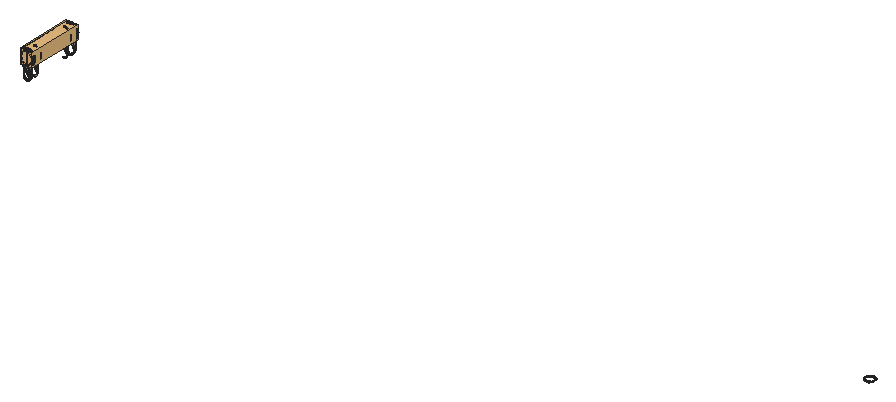
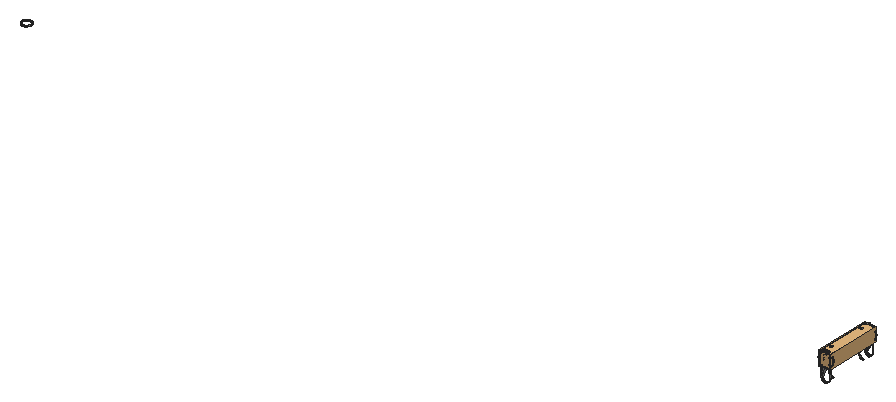
# SketchUp Ruby script. Lengths in inches.
U = 1.inch
M = Sketchup.active_model
def pt(a) = Geom::Point3d.new(a.map { |v| v * U })
def face(e, loops, mat)
  f = e.add_face(loops[0].map { |a| pt(a) })
  loops[1..].each { |l| e.add_face(l.map { |a| pt(a) }).erase! }
  f.material = f.back_material = mat if mat
  f
end
# faces: each face lists its corners as indices into pts; further lists are holes
def faces(e, pts, list, mat = nil) = list.each { |f| face(e, (f[0].is_a?(Array) ? f : [f]).map { |l| l.map { |i| pts[i] } }, mat) }
# xy, xz, yz: faces in a plane at the given z, y or x. An outline is a flat list of corners, or four numbers for a rectangle; further outlines are holes
def ring(l) = l.size == 4 ? [[l[0], l[1]], [l[2], l[1]], [l[2], l[3]], [l[0], l[3]]] : l.each_slice(2).to_a
def flat(e, list, mat, &to3) = list.each { |f| face(e, (f[0].is_a?(Array) ? f : [f]).map { |l| ring(l).map { |u, v| to3.(u, v) } }, mat) }
def xy(e, z, list, mat = nil) = flat(e, list, mat) { |x, y| [x, y, z] }
def xz(e, y, list, mat = nil) = flat(e, list, mat) { |x, z| [x, y, z] }
def yz(e, x, list, mat = nil) = flat(e, list, mat) { |y, z| [x, y, z] }
def lines(e, pts, list) = list.each { |a, b| e.add_line(pt(pts[a]), pt(pts[b])) }
# prism: a flat outline (further loops are holes) pulled along v
def prism(e, loops, v, mat = nil)
  f = face(e, loops, mat); d = Geom::Vector3d.new(v.map { |x| x * U })
  f.pushpull(f.normal.samedirection?(d) ? d.length : -d.length)
end
def box(e, o, s, mat = nil) = prism(e, [[o, [o[0] + s[0], o[1], o[2]], [o[0] + s[0], o[1] + s[1], o[2]], [o[0], o[1] + s[1], o[2]]]], [0, 0, s[2]], mat)
def at(x, y, z, deg = 0) = Geom::Transformation.translation(pt([x, y, z])) * Geom::Transformation.rotation(ORIGIN, Z_AXIS, deg.degrees)
def axes(o, x, y, z) = Geom::Transformation.new([*x, 0, *y, 0, *z, 0, *pt(o).to_a, 1])
def part(name) = M.definitions.add(name)
# library, detail: a bought-in or finely detailed component or shape, given as its bounding box
def library(name, o, s) = part(name).tap { |d| box(d.entities, o, s) }
def detail(e, o, s) = box(e.add_group.entities, o, s)
def put(e, d, t, mat = nil) = e.add_instance(d, t).tap { |i| i.material = mat if mat }
def group(e, t, mat = nil) = e.add_group.tap { |g| g.transformation = t; g.material = mat if mat }.entities
root = M.entities
M.materials.add("Material \#1").color = [140, 140, 140]
c1 = library("3DGeom~12_Defintion",[-95.68,-755.75,-830.03],[191.36,191.37,1000])
c2 = part("3DGeom~10_Defintion")
yz(c2.entities,-68.96,[[-797.08,-844.83,-797.08,-827.59,-922.41,-827.59],[-922.41,-844.83,-797.08,-844.83,-922.41,-827.59]],"Material \#1")
yz(c2.entities,68.97,[[-922.41,-844.83,-797.08,-827.59,-797.08,-844.83],[-922.41,-844.83,-922.41,-827.59,-797.08,-827.59],[-797.08,137.93,-922.41,155.17,-797.08,155.17],[-922.41,137.93,-922.41,155.17,-797.08,137.93]],"Material \#1")
p = [[-15.8,-989.55,-844.83],[-15.8,-989.55,-827.59],[0,-991.38,-827.59],[0,-991.38,-844.83],[15.8,-989.55,-827.59],[15.8,-989.55,-844.83],
  [-30.32,-984.36,-844.83],[-30.32,-984.36,-827.59],[30.31,-984.36,-827.59],[30.31,-984.36,-844.83],[-43.12,-976.21,-844.83],[-43.12,-976.21,-827.59],
  [43.12,-976.21,-827.59],[43.12,-976.21,-844.83],[-53.81,-965.53,-844.83],[-53.81,-965.53,-827.59],[53.8,-965.53,-827.59],[53.8,-965.53,-844.83],
  [-61.95,-952.73,-844.83],[-61.95,-952.73,-827.59],[53.8,-965.53,-827.59],[61.95,-952.73,-827.59],[61.95,-952.73,-844.83],[-67.15,-938.21,-844.83],
  [-67.15,-938.21,-827.59],[67.14,-938.21,-827.59],[67.14,-938.21,-844.83],[-68.96,-922.41,-844.83],[-68.96,-922.41,-827.59],[67.14,-938.21,-827.59],
  [68.97,-922.41,-827.59],[68.97,-922.41,-844.83],[-69.1,-794.86,-844.83],[-69.1,-794.86,-827.59],[-68.96,-797.08,-827.59],[-68.96,-797.08,-844.83],
  [68.97,-797.08,-844.83],[68.97,-797.08,-827.59],[69.11,-794.71,-827.59],[69.11,-794.71,-844.83],[-69.48,-792.73,-844.83],[-69.48,-792.73,-827.59],
  [69.53,-792.51,-827.59],[69.53,-792.51,-844.83],[-70.14,-790.6875,-844.83],[-70.14,-790.6875,-827.59],[70.24,-790.48,-827.59],[70.24,-790.48,-844.83],
  [-71.08,-788.73,-844.83],[-71.08,-788.73,-827.59],[71.22,-788.57,-827.59],[71.22,-788.57,-844.83],[-72.32,-786.86,-844.83],[-72.32,-786.86,-827.59],
  [72.47,-786.78,-827.59],[72.47,-786.78,-844.83],[-73.8,-785.17,-844.83],[-73.8,-785.17,-827.59],[74,-785.04,-827.59],[74,-785.04,-844.83],
  [-75.96,-783.21,-844.83],[-75.96,-783.21,-827.59],[74,-785.04,-827.59],[75.76,-783.39,-827.59],[75.76,-783.39,-844.83],[86.625,-772.95,-827.59],
  [86.61,-772.96,-844.83],[-86.89,-773.25,-844.83],[-86.89,-773.25,-827.59],[-75.96,-783.21,-844.83],[-96.66,-761.8,-844.83],[-96.66,-761.8,-827.59],
  [86.625,-772.95,-827.59],[86.63,-772.94,-844.83],[86.61,-772.96,-844.83],[86.625,-772.95,-827.59],[86.62,-772.95,-827.59],[86.62,-772.95,-827.59],
  [96.31,-761.375,-827.59],[96.31,-761.375,-844.83],[86.63,-772.94,-844.83],[86.625,-772.95,-827.59],[86.62,-772.95,-827.59],[-104.96,-749.18,-844.83],
  [-104.96,-749.18,-827.59],[-96.66,-761.8,-827.59],[-96.66,-761.8,-844.83],[96.31,-761.375,-827.59],[104.62,-748.77,-827.59],[104.62,-748.77,-844.83],
  [-111.64,-735.52,-844.83],[-111.64,-735.52,-827.59],[111.39,-735.21,-827.59],[111.39,-735.21,-844.83],[-116.49,-721.23,-844.83],[-116.49,-721.23,-827.59],
  [116.4375,-720.78,-827.59],[116.4375,-720.78,-844.83],[-119.64,-705.62,-844.83],[-119.64,-705.62,-827.59],[119.6,-705.57,-827.59],[119.6,-705.57,-844.83],
  [-120.6875,-689.65,-844.83],[-120.6875,-689.65,-827.59],[120.69,-689.65,-827.59],[120.69,-689.65,-844.83],[-117.5,-662,-844.83],[-117.5,-662,-827.59],
  [117.5,-662,-827.59],[117.5,-662,-844.83],[-108.41,-636.61,-844.83],[-108.41,-636.61,-827.59],[117.5,-662,-844.83],[108.41,-636.61,-827.59],
  [108.41,-636.61,-844.83],[-93.91,-613.95,-844.83],[-93.91,-613.95,-827.59],[-108.41,-636.61,-827.59],[108.41,-636.61,-844.83],[94.16,-614.19,-827.59],
  [94.16,-614.19,-844.83],[94.16,-614.19,-827.59],[75.46,-595.5,-827.59],[75.46,-595.5,-844.83],[-75.46,-595.5,-844.83],[-75.46,-595.5,-827.59],
  [-93.91,-613.95,-827.59],[-93.91,-613.95,-827.59],[-93.91,-613.95,-844.83],[-53.05,-581.24,-844.83],[-53.05,-581.24,-827.59],[-75.46,-595.5,-827.59],
  [-75.46,-595.5,-844.83],[53.05,-581.24,-827.59],[53.05,-581.24,-844.83],[-27.65,-572.16,-844.83],[-27.65,-572.16,-827.59],[-53.05,-581.24,-827.59],
  [-53.05,-581.24,-844.83],[27.66,-572.16,-827.59],[27.66,-572.16,-844.83],[0,-568.97,-844.83],[0,-568.97,-827.59],[-27.65,-572.16,-827.59],
  [-27.65,-572.16,-844.83],[0,-568.97,-844.83],[-15.8,-989.55,155.17],[0,-991.38,155.17],[0,-991.38,137.93],[-15.8,-989.55,137.93],
  [15.8,-989.55,155.17],[15.8,-989.55,137.93],[-30.32,-984.36,155.17],[-30.32,-984.36,137.93],[30.31,-984.36,155.17],[30.31,-984.36,137.93],
  [-43.125,-976.22,155.17],[-43.125,-976.22,137.93],[43.12,-976.22,155.17],[43.12,-976.22,137.93],[-53.81,-965.53,155.17],[-53.81,-965.53,137.93],
  [53.8,-965.53,155.17],[53.8,-965.53,137.93],[-61.96,-952.73,155.17],[-61.95,-952.73,137.93],[61.95,-952.73,155.17],[61.95,-952.73,137.93],
  [53.8,-965.53,137.93],[-67.15,-938.21,155.17],[-67.15,-938.21,137.93],[67.14,-938.21,155.17],[67.14,-938.21,137.93],[-68.96,-922.41,155.17],
  [-68.96,-922.41,137.93],[68.97,-922.41,155.17],[68.97,-922.41,137.93],[67.14,-938.21,137.93],[-68.97,-797.08,155.17],[-68.97,-797.08,137.93],
  [-69.1,-794.86,155.17],[-69.1,-794.86,137.93],[68.97,-797.08,155.17],[69.11,-794.71,155.17],[69.11,-794.71,137.93],[68.97,-797.08,137.93],
  [-69.48,-792.73,155.17],[-69.48,-792.73,137.93],[69.53,-792.51,155.17],[69.53,-792.51,137.93],[-70.14,-790.6875,155.17],[-70.14,-790.6875,137.93],
  [70.24,-790.48,155.17],[70.24,-790.48,137.93],[-71.08,-788.73,155.17],[-71.08,-788.73,137.93],[71.22,-788.57,155.17],[71.22,-788.57,137.93],
  [-72.32,-786.86,155.17],[-72.32,-786.86,137.93],[72.47,-786.78,155.17],[72.47,-786.78,137.93],[-73.8,-785.17,155.17],[-73.8,-785.17,137.93],
  [74,-785.04,155.17],[74,-785.04,137.93],[-75.96,-783.21,155.17],[-75.96,-783.21,137.93],[75.76,-783.39,155.17],[75.76,-783.39,137.93],
  [74,-785.04,137.93],[86.61,-772.96,155.17],[86.625,-772.95,137.93],[-86.88,-773.25,155.17],[-75.96,-783.21,155.17],[-86.88,-773.25,137.93],
  [-96.66,-761.8,155.17],[-96.66,-761.8,137.93],[86.63,-772.94,155.17],[86.625,-772.95,137.93],[86.61,-772.96,155.17],[86.62,-772.95,137.93],
  [86.625,-772.95,137.93],[96.31,-761.375,155.17],[96.31,-761.375,137.93],[86.62,-772.95,137.93],[86.63,-772.94,155.17],[86.62,-772.95,137.93],
  [86.625,-772.95,137.93],[-104.96,-749.18,155.17],[-96.66,-761.8,155.17],[-96.66,-761.8,137.93],[-104.96,-749.18,137.93],[104.62,-748.77,155.17],
  [104.62,-748.77,137.93],[96.31,-761.375,137.93],[-111.64,-735.52,155.17],[-111.64,-735.52,137.93],[111.39,-735.21,155.17],[111.39,-735.21,137.93],
  [-116.49,-721.23,155.17],[-116.49,-721.23,137.93],[116.4375,-720.78,155.17],[116.4375,-720.78,137.93],[-119.64,-705.62,155.17],[-119.64,-705.62,137.93],
  [119.6,-705.57,155.17],[119.6,-705.57,137.93],[-120.6875,-689.65,155.17],[-120.6875,-689.65,137.93],[120.69,-689.65,155.17],[120.69,-689.65,137.93],
  [-117.5,-662,155.17],[-117.5,-662,137.93],[117.5,-662,155.17],[117.5,-662,137.93],[-108.41,-636.61,155.17],[-108.41,-636.61,137.93],
  [117.5,-662,155.17],[108.41,-636.61,155.17],[108.41,-636.61,137.93],[-93.91,-613.95,155.17],[-108.41,-636.61,137.93],[-93.91,-613.95,137.93],
  [108.41,-636.61,155.17],[94.16,-614.19,155.17],[94.16,-614.19,137.93],[75.46,-595.5,155.17],[75.46,-595.5,137.93],[94.16,-614.19,137.93],
  [-75.46,-595.5,155.17],[-93.91,-613.95,155.17],[-93.91,-613.95,137.93],[-75.46,-595.5,137.93],[-53.05,-581.24,155.17],[-75.46,-595.5,155.17],
  [-75.46,-595.5,137.93],[-53.05,-581.24,137.93],[53.05,-581.24,155.17],[53.05,-581.24,137.93],[-27.65,-572.16,155.17],[-53.05,-581.24,155.17],
  [-53.05,-581.24,137.93],[-27.65,-572.16,137.93],[27.65,-572.16,155.17],[27.65,-572.16,137.93],[0,-568.97,155.17],[-27.65,-572.16,155.17],
  [-27.65,-572.16,137.93],[0,-568.97,137.93],[0,-568.97,155.17]]
faces(c2.entities,p,[[0,1,2],[2,3,0],[3,2,4],[4,5,3],[6,7,1],[1,0,6],[5,4,8],[8,9,5],
  [10,11,7],[7,6,10],[9,8,12],[12,13,9],[14,15,11],[11,10,14],[13,12,16],[16,17,13],
  [18,19,15],[15,14,18],[17,20,21],[21,22,17],[23,24,19],[19,18,23],[22,21,25],[25,26,22],
  [27,28,24],[24,23,27],[26,29,30],[30,31,26],[32,33,34],[34,35,32],[36,37,38],[38,39,36],
  [40,41,33],[33,32,40],[39,38,42],[42,43,39],[44,45,41],[41,40,44],[43,42,46],[46,47,43],
  [48,49,45],[45,44,48],[47,46,50],[50,51,47],[52,53,49],[49,48,52],[51,50,54],[54,55,51],
  [56,57,53],[53,52,56],[55,54,58],[58,59,55],[60,61,57],[57,56,60],[59,62,63],[63,64,59],
  [64,63,65],[65,66,64],[67,68,61],[61,69,67],[70,71,68],[68,67,70],[72,73,66],[74,75,76],
  [73,77,78],[78,79,73],[80,81,82],[83,84,85],[85,86,83],[79,87,88],[88,89,79],[90,91,84],
  [84,83,90],[89,88,92],[92,93,89],[94,95,91],[91,90,94],[93,92,96],[96,97,93],[98,99,95],
  [95,94,98],[97,96,100],[100,101,97],[102,103,99],[99,98,102],[101,100,104],[104,105,101],[106,107,103],
  [103,102,106],[105,104,108],[108,109,105],[110,111,107],[107,106,110],[112,108,113],[113,114,112],[115,116,117],
  [117,110,115],[118,113,119],[119,120,118],[120,121,122],[122,123,120],[124,125,126],[127,128,124],[129,130,131],
  [131,132,129],[123,122,133],[133,134,123],[135,136,137],[137,138,135],[134,133,139],[139,140,134],[141,142,143],
  [143,144,141],[140,139,142],[142,145,140],[146,147,148],[148,149,146],[147,150,151],[151,148,147],[152,146,149],
  [149,153,152],[150,154,155],[155,151,150],[156,152,153],[153,157,156],[154,158,159],[159,155,154],[160,156,157],
  [157,161,160],[158,162,163],[163,159,158],[164,160,161],[161,165,164],[162,166,167],[167,168,162],[169,164,165],
  [165,170,169],[166,171,172],[172,167,166],[173,169,170],[170,174,173],[171,175,176],[176,177,171],[178,173,174],
  [174,179,178],[180,178,179],[179,181,180],[182,183,184],[184,185,182],[186,180,181],[181,187,186],[183,188,189],
  [189,184,183],[190,186,187],[187,191,190],[188,192,193],[193,189,188],[194,190,191],[191,195,194],[192,196,197],
  [197,193,192],[198,194,195],[195,199,198],[196,200,201],[201,197,196],[202,198,199],[199,203,202],[200,204,205],
  [205,201,200],[206,202,203],[203,207,206],[204,208,209],[209,210,204],[208,211,212],[212,209,208],[213,214,207],
  [207,215,213],[216,213,215],[215,217,216],[211,218,219],[220,221,222],[218,223,224],[224,225,218],[226,227,228],
  [229,230,231],[231,232,229],[223,233,234],[234,235,223],[236,229,232],[232,237,236],[233,238,239],[239,234,233],
  [240,236,237],[237,241,240],[238,242,243],[243,239,238],[244,240,241],[241,245,244],[242,246,247],[247,243,242],
  [248,244,245],[245,249,248],[246,250,251],[251,247,246],[252,248,249],[249,253,252],[250,254,255],[255,251,250],
  [256,252,253],[253,257,256],[258,259,260],[260,255,258],[261,256,262],[262,263,261],[264,265,266],[266,260,264],
  [265,267,268],[268,269,265],[270,271,272],[272,273,270],[274,275,276],[276,277,274],[267,278,279],[279,268,267],
  [280,281,282],[282,283,280],[278,284,285],[285,279,278],[286,287,288],[288,289,286],[284,290,289],[289,285,284]],"Material \#1")
c3 = library("3DGeom~13_Defintion",[-84.91,-744.98,-830.03],[169.82,169.83,1000])
xy(root,49.893,[[128.435,116.314,128.381,116.332,128.389,116.346],[128.435,116.314,128.389,116.346,128.4375,116.329],[128.435,116.314,128.4375,116.329,128.492,116.314],[128.492,116.314,128.4375,116.329,128.489,116.329],[128.492,116.314,128.489,116.329,128.545,116.332],
  [128.489,116.329,128.537,116.346,128.545,116.332],[128.381,116.332,128.337,116.367,128.35,116.377],[128.381,116.332,128.35,116.377,128.389,116.346],[128.545,116.332,128.537,116.346,128.589,116.367],[128.537,116.346,128.576,116.377,128.589,116.367],
  [128.337,116.367,128.309,116.413,128.324,116.418],[128.337,116.367,128.324,116.418,128.35,116.377],[128.589,116.367,128.576,116.377,128.617,116.413],[128.576,116.377,128.602,116.418,128.617,116.413],[128.309,116.413,128.299,116.465,128.315,116.465],
  [128.309,116.413,128.315,116.465,128.324,116.418],[128.617,116.413,128.602,116.418,128.627,116.465],[128.602,116.418,128.611,116.465,128.627,116.465],[128.299,116.465,128.309,116.518,128.324,116.513],[128.299,116.465,128.324,116.513,128.315,116.465],
  [128.611,116.465,128.602,116.513,128.617,116.518],[128.611,116.465,128.617,116.518,128.627,116.465],[128.324,116.513,128.309,116.518,128.35,116.554],[128.602,116.513,128.576,116.554,128.589,116.564],[128.602,116.513,128.589,116.564,128.617,116.518],
  [128.309,116.518,128.337,116.564,128.35,116.554],[128.35,116.554,128.337,116.564,128.389,116.585],[128.576,116.554,128.537,116.585,128.545,116.598],[128.576,116.554,128.545,116.598,128.589,116.564],[128.337,116.564,128.381,116.598,128.389,116.585],
  [128.389,116.585,128.381,116.598,128.4375,116.601],[128.537,116.585,128.489,116.601,128.492,116.616],[128.537,116.585,128.492,116.616,128.545,116.598],[128.381,116.598,128.435,116.616,128.4375,116.601],[128.4375,116.601,128.435,116.616,128.489,116.601],
  [128.489,116.601,128.435,116.616,128.492,116.616]],"Material \#1")
xy(root,49.908,[[128.435,116.314,128.4375,116.329,128.381,116.332],[128.435,116.314,128.489,116.329,128.4375,116.329],[128.435,116.314,128.492,116.314,128.489,116.329],[128.492,116.314,128.537,116.346,128.489,116.329],[128.492,116.314,128.545,116.332,128.537,116.346],
  [128.4375,116.329,128.389,116.346,128.381,116.332],[128.381,116.332,128.389,116.346,128.337,116.367],[128.545,116.332,128.576,116.377,128.537,116.346],[128.545,116.332,128.589,116.367,128.576,116.377],[128.389,116.346,128.35,116.377,128.337,116.367],
  [128.337,116.367,128.35,116.377,128.309,116.413],[128.589,116.367,128.602,116.418,128.576,116.377],[128.589,116.367,128.617,116.413,128.602,116.418],[128.35,116.377,128.324,116.418,128.309,116.413],[128.309,116.413,128.324,116.418,128.299,116.465],
  [128.617,116.413,128.611,116.465,128.602,116.418],[128.617,116.413,128.627,116.465,128.611,116.465],[128.324,116.418,128.315,116.465,128.299,116.465],[128.299,116.465,128.315,116.465,128.309,116.518],[128.315,116.465,128.324,116.513,128.309,116.518],
  [128.611,116.465,128.627,116.465,128.602,116.513],[128.627,116.465,128.617,116.518,128.602,116.513],[128.324,116.513,128.337,116.564,128.309,116.518],[128.324,116.513,128.35,116.554,128.337,116.564],[128.602,116.513,128.617,116.518,128.576,116.554],
  [128.617,116.518,128.589,116.564,128.576,116.554],[128.35,116.554,128.381,116.598,128.337,116.564],[128.35,116.554,128.389,116.585,128.381,116.598],[128.576,116.554,128.589,116.564,128.537,116.585],[128.589,116.564,128.545,116.598,128.537,116.585],
  [128.389,116.585,128.435,116.616,128.381,116.598],[128.389,116.585,128.4375,116.601,128.435,116.616],[128.537,116.585,128.545,116.598,128.489,116.601],[128.545,116.598,128.492,116.616,128.489,116.601],[128.4375,116.601,128.492,116.616,128.435,116.616],
  [128.4375,116.601,128.489,116.601,128.492,116.616]],"Material \#1")
xy(root,49.922,[[101.384,115.812,101.384,116.097,101.412,116.097],[101.384,115.812,101.412,116.097,101.412,115.812],[101.384,117.386,101.384,117.671,101.412,117.386],[101.412,117.386,101.384,117.671,101.412,117.671]],"Material \#1")
xy(root,50.231,[[101.369,115.812,101.417,115.812,101.369,116.097],[101.417,115.812,101.417,116.097,101.369,116.097],[101.369,117.386,101.417,117.386,101.417,117.671]],"Material \#1")
xz(root,115.812,[[101.393,49.869,101.347,49.876,101.393,49.877],[101.393,49.869,101.393,49.877,101.436,49.884],[101.393,49.869,101.436,49.884,101.438,49.876],[101.347,49.876,101.305,49.897,101.349,49.884],[101.347,49.876,101.349,49.884,101.393,49.877],
  [101.438,49.876,101.436,49.884,101.477,49.904],[101.438,49.876,101.477,49.904,101.481,49.897],[101.349,49.884,101.305,49.897,101.308,49.904],[101.305,49.897,101.269,49.93,101.308,49.904],[101.481,49.897,101.477,49.904,101.512,49.936],
  [101.481,49.897,101.512,49.936,101.517,49.93],[101.308,49.904,101.269,49.93,101.273,49.936],[101.269,49.93,101.241,49.973,101.273,49.936],[101.517,49.93,101.512,49.936,101.539,49.977],[101.517,49.93,101.539,49.977,101.545,49.973],
  [101.273,49.936,101.241,49.973,101.247,49.977],[101.241,49.973,101.223,50.023,101.247,49.977],[101.545,49.973,101.539,49.977,101.556,50.025],[101.545,49.973,101.556,50.025,101.562,50.023],[101.247,49.977,101.223,50.023,101.23,50.025],
  [101.223,50.023,101.217,50.076,101.23,50.025],[101.562,50.023,101.556,50.025,101.562,50.076],[101.562,50.023,101.562,50.076,101.568,50.076],[101.23,50.025,101.217,50.076,101.224,50.076],[101.217,50.076,101.223,50.13,101.224,50.076],
  [101.224,50.076,101.223,50.13,101.23,50.128],[101.562,50.076,101.556,50.128,101.568,50.076],[101.568,50.076,101.556,50.128,101.562,50.13],[101.23,50.128,101.223,50.13,101.241,50.18],[101.23,50.128,101.241,50.18,101.247,50.176],
  [101.556,50.128,101.539,50.176,101.562,50.13],[101.562,50.13,101.539,50.176,101.545,50.18],[101.247,50.176,101.241,50.18,101.269,50.223],[101.247,50.176,101.269,50.223,101.273,50.217],[101.539,50.176,101.512,50.217,101.545,50.18],
  [101.545,50.18,101.512,50.217,101.517,50.223],[101.273,50.217,101.269,50.223,101.305,50.256],[101.273,50.217,101.305,50.256,101.308,50.249],[101.512,50.217,101.477,50.249,101.517,50.223],[101.517,50.223,101.477,50.249,101.481,50.256],
  [101.308,50.249,101.305,50.256,101.347,50.277],[101.308,50.249,101.347,50.277,101.349,50.269],[101.477,50.249,101.436,50.269,101.481,50.256],[101.481,50.256,101.436,50.269,101.438,50.277],[101.349,50.269,101.347,50.277,101.393,50.284],
  [101.349,50.269,101.393,50.284,101.393,50.276],[101.436,50.269,101.393,50.276,101.438,50.277],[101.393,50.276,101.393,50.284,101.438,50.277]],"Material \#1")
xz(root,115.821,[[101.393,49.407,101.448,49.421,101.421,49.41],[101.393,49.407,101.49,49.462,101.448,49.421],[101.448,49.421,101.49,49.462,101.471,49.439],[101.49,49.462,101.239,49.931,101.27,49.895],[101.49,49.462,101.265,49.852,101.263,49.858],
  [101.49,49.462,101.267,49.847,101.265,49.852],[101.49,49.462,101.268,49.841,101.267,49.847],[101.49,49.462,101.27,49.895,101.306,49.868],[101.49,49.462,101.348,49.85,101.393,49.844],[101.49,49.462,101.393,49.844,101.517,49.554],
  [101.49,49.462,101.514,49.52,101.505,49.489],[101.49,49.462,101.517,49.554,101.514,49.52],[101.517,49.554,101.393,49.844,101.438,49.85],[101.517,49.554,101.438,49.85,101.479,49.868],[101.517,49.554,101.479,49.868,101.516,49.895],
  [101.517,49.554,101.516,49.895,101.517,49.835],[101.517,49.835,101.516,49.895,101.519,49.848],[101.517,49.835,101.519,49.848,101.518,49.842],[101.519,49.848,101.516,49.895,101.546,49.931],[101.519,49.848,101.523,49.858,101.52,49.853],
  [101.519,49.848,101.546,49.931,101.523,49.858],[101.523,49.858,101.546,49.931,101.57,49.974],[101.523,49.858,101.57,49.974,101.614,50.042],[101.523,49.858,101.614,50.042,101.525,49.863],[101.525,49.863,101.614,50.042,101.529,49.867],
  [101.529,49.867,101.571,49.92,101.533,49.872],[101.529,49.867,101.614,50.042,101.571,49.92],[101.533,49.872,101.571,49.92,101.553,49.895],[101.571,49.92,101.599,49.977,101.586,49.947],[101.571,49.92,101.614,50.042,101.599,49.977],
  [101.57,49.974,101.584,50.023,101.614,50.042],[101.599,49.977,101.614,50.042,101.608,50.009],[101.584,50.023,101.59,50.076,101.614,50.042],[101.614,50.042,101.567,50.241,101.61,50.137],[101.614,50.042,101.57,50.179,101.567,50.241],
  [101.614,50.042,101.584,50.13,101.57,50.179],[101.614,50.042,101.59,50.076,101.584,50.13],[101.614,50.042,101.61,50.137,101.616,50.076],[101.61,50.137,101.567,50.241,101.593,50.192],[101.57,50.179,101.546,50.222,101.567,50.241],
  [101.546,50.222,101.516,50.258,101.567,50.241],[101.567,50.241,101.393,50.34,101.491,50.313],[101.567,50.241,101.479,50.285,101.393,50.34],[101.567,50.241,101.516,50.258,101.479,50.285],[101.567,50.241,101.491,50.313,101.532,50.282],
  [101.479,50.285,101.438,50.303,101.393,50.34],[101.438,50.303,101.393,50.309,101.393,50.34],[101.491,50.313,101.393,50.34,101.444,50.333]],"Material \#1")
xz(root,116.128,[[101.393,49.407,101.421,49.41,101.448,49.421],[101.338,49.421,101.448,49.421,101.514,49.52],[101.448,49.421,101.471,49.439,101.49,49.462],[101.448,49.421,101.49,49.462,101.514,49.52],[101.49,49.462,101.505,49.489,101.514,49.52],
  [101.514,49.52,101.517,49.554,101.263,49.858],[101.517,49.554,101.393,49.844,101.348,49.85],[101.517,49.554,101.438,49.85,101.393,49.844],[101.517,49.554,101.517,49.835,101.438,49.85],[101.517,49.835,101.519,49.848,101.438,49.85],
  [101.517,49.835,101.518,49.842,101.519,49.848],[101.519,49.848,101.523,49.858,101.438,49.85],[101.519,49.848,101.52,49.853,101.523,49.858],[101.438,49.85,101.523,49.858,101.479,49.868],[101.523,49.858,101.516,49.895,101.479,49.868],
  [101.523,49.858,101.546,49.931,101.516,49.895],[101.523,49.858,101.525,49.863,101.614,50.042],[101.523,49.858,101.614,50.042,101.546,49.931],[101.525,49.863,101.529,49.867,101.614,50.042],[101.529,49.867,101.533,49.872,101.571,49.92],
  [101.529,49.867,101.571,49.92,101.614,50.042],[101.533,49.872,101.553,49.895,101.571,49.92],[101.571,49.92,101.586,49.947,101.599,49.977],[101.571,49.92,101.599,49.977,101.614,50.042],[101.546,49.931,101.614,50.042,101.57,49.974],
  [101.57,49.974,101.614,50.042,101.584,50.023],[101.599,49.977,101.608,50.009,101.614,50.042],[101.584,50.023,101.614,50.042,101.59,50.076],[101.614,50.042,101.567,50.241,101.584,50.13],[101.614,50.042,101.61,50.137,101.567,50.241],
  [101.614,50.042,101.584,50.13,101.59,50.076],[101.614,50.042,101.616,50.076,101.61,50.137],[101.584,50.13,101.567,50.241,101.57,50.179],[101.61,50.137,101.593,50.192,101.567,50.241],[101.57,50.179,101.567,50.241,101.546,50.222],
  [101.546,50.222,101.567,50.241,101.516,50.258],[101.567,50.241,101.393,50.34,101.479,50.285],[101.567,50.241,101.491,50.313,101.393,50.34],[101.567,50.241,101.479,50.285,101.516,50.258],[101.567,50.241,101.532,50.282,101.491,50.313],
  [101.479,50.285,101.393,50.34,101.438,50.303],[101.438,50.303,101.393,50.34,101.393,50.309],[101.491,50.313,101.444,50.333,101.393,50.34]],"Material \#1")
xz(root,117.355,[[101.393,49.407,101.448,49.421,101.421,49.41],[101.338,49.421,101.514,49.52,101.448,49.421],[101.448,49.421,101.49,49.462,101.471,49.439],[101.448,49.421,101.514,49.52,101.49,49.462],[101.49,49.462,101.514,49.52,101.505,49.489],
  [101.514,49.52,101.263,49.858,101.517,49.554],[101.517,49.554,101.348,49.85,101.393,49.844],[101.517,49.554,101.393,49.844,101.438,49.85],[101.517,49.554,101.438,49.85,101.517,49.835],[101.517,49.835,101.438,49.85,101.519,49.848],
  [101.517,49.835,101.519,49.848,101.518,49.842],[101.519,49.848,101.438,49.85,101.523,49.858],[101.519,49.848,101.523,49.858,101.52,49.853],[101.438,49.85,101.479,49.868,101.523,49.858],[101.523,49.858,101.479,49.868,101.516,49.895],
  [101.523,49.858,101.516,49.895,101.546,49.931],[101.523,49.858,101.546,49.931,101.614,50.042],[101.523,49.858,101.614,50.042,101.525,49.863],[101.525,49.863,101.614,50.042,101.529,49.867],[101.529,49.867,101.571,49.92,101.533,49.872],
  [101.529,49.867,101.614,50.042,101.571,49.92],[101.533,49.872,101.571,49.92,101.553,49.895],[101.571,49.92,101.599,49.977,101.586,49.947],[101.571,49.92,101.614,50.042,101.599,49.977],[101.546,49.931,101.57,49.974,101.614,50.042],
  [101.57,49.974,101.584,50.023,101.614,50.042],[101.599,49.977,101.614,50.042,101.608,50.009],[101.584,50.023,101.59,50.076,101.614,50.042],[101.614,50.042,101.567,50.241,101.61,50.137],[101.614,50.042,101.584,50.13,101.567,50.241],
  [101.614,50.042,101.59,50.076,101.584,50.13],[101.614,50.042,101.61,50.137,101.616,50.076],[101.584,50.13,101.57,50.179,101.567,50.241],[101.61,50.137,101.567,50.241,101.593,50.192],[101.57,50.179,101.546,50.222,101.567,50.241],
  [101.546,50.222,101.516,50.258,101.567,50.241],[101.567,50.241,101.393,50.34,101.491,50.313],[101.567,50.241,101.479,50.285,101.393,50.34],[101.567,50.241,101.516,50.258,101.479,50.285],[101.567,50.241,101.491,50.313,101.532,50.282],
  [101.479,50.285,101.438,50.303,101.393,50.34],[101.438,50.303,101.393,50.309,101.393,50.34],[101.491,50.313,101.393,50.34,101.444,50.333]],"Material \#1")
xz(root,117.601,[[101.393,49.844,101.393,49.852,101.342,49.852],[101.393,49.844,101.442,49.86,101.393,49.852],[101.393,49.844,101.444,49.852,101.442,49.86],[101.342,49.852,101.344,49.86,101.294,49.875],[101.342,49.852,101.393,49.852,101.344,49.86],
  [101.444,49.852,101.488,49.882,101.442,49.86],[101.444,49.852,101.491,49.875,101.488,49.882],[101.344,49.86,101.298,49.882,101.294,49.875],[101.294,49.875,101.298,49.882,101.254,49.912],[101.491,49.875,101.527,49.918,101.488,49.882],
  [101.491,49.875,101.532,49.912,101.527,49.918],[101.298,49.882,101.258,49.918,101.254,49.912],[101.254,49.912,101.258,49.918,101.222,49.96],[101.532,49.912,101.558,49.964,101.527,49.918],[101.532,49.912,101.563,49.96,101.558,49.964],
  [101.258,49.918,101.228,49.964,101.222,49.96],[101.222,49.96,101.228,49.964,101.203,50.016],[101.563,49.96,101.577,50.018,101.558,49.964],[101.563,49.96,101.583,50.016,101.577,50.018],[101.228,49.964,101.209,50.018,101.203,50.016],
  [101.203,50.016,101.209,50.018,101.196,50.076],[101.583,50.016,101.583,50.076,101.577,50.018],[101.583,50.016,101.59,50.076,101.583,50.076],[101.209,50.018,101.203,50.076,101.196,50.076],[101.196,50.076,101.203,50.076,101.203,50.137],
  [101.203,50.076,101.209,50.135,101.203,50.137],[101.583,50.076,101.59,50.076,101.577,50.135],[101.59,50.076,101.583,50.137,101.577,50.135],[101.209,50.135,101.222,50.193,101.203,50.137],[101.209,50.135,101.228,50.189,101.222,50.193],
  [101.577,50.135,101.583,50.137,101.558,50.189],[101.583,50.137,101.563,50.193,101.558,50.189],[101.228,50.189,101.254,50.241,101.222,50.193],[101.228,50.189,101.258,50.235,101.254,50.241],[101.558,50.189,101.563,50.193,101.527,50.235],
  [101.563,50.193,101.532,50.241,101.527,50.235],[101.258,50.235,101.294,50.278,101.254,50.241],[101.258,50.235,101.298,50.271,101.294,50.278],[101.527,50.235,101.532,50.241,101.488,50.271],[101.532,50.241,101.491,50.278,101.488,50.271],
  [101.298,50.271,101.342,50.301,101.294,50.278],[101.298,50.271,101.344,50.293,101.342,50.301],[101.488,50.271,101.491,50.278,101.442,50.293],[101.491,50.278,101.444,50.301,101.442,50.293],[101.344,50.293,101.393,50.309,101.342,50.301],
  [101.344,50.293,101.393,50.301,101.393,50.309],[101.442,50.293,101.444,50.301,101.393,50.301],[101.393,50.301,101.444,50.301,101.393,50.309]],"Material \#1")
xz(root,117.662,[[101.393,49.407,101.421,49.41,101.448,49.421],[101.393,49.407,101.448,49.421,101.49,49.462],[101.448,49.421,101.471,49.439,101.49,49.462],[101.49,49.462,101.393,49.844,101.348,49.85],[101.49,49.462,101.517,49.554,101.393,49.844],
  [101.49,49.462,101.505,49.489,101.514,49.52],[101.49,49.462,101.514,49.52,101.517,49.554],[101.517,49.554,101.438,49.85,101.393,49.844],[101.517,49.554,101.479,49.868,101.438,49.85],[101.517,49.554,101.516,49.895,101.479,49.868],
  [101.517,49.554,101.517,49.835,101.516,49.895],[101.517,49.835,101.519,49.848,101.516,49.895],[101.517,49.835,101.518,49.842,101.519,49.848],[101.519,49.848,101.546,49.931,101.516,49.895],[101.519,49.848,101.52,49.853,101.523,49.858],
  [101.519,49.848,101.523,49.858,101.546,49.931],[101.523,49.858,101.525,49.863,101.614,50.042],[101.523,49.858,101.57,49.974,101.546,49.931],[101.523,49.858,101.614,50.042,101.57,49.974],[101.525,49.863,101.529,49.867,101.614,50.042],
  [101.529,49.867,101.533,49.872,101.571,49.92],[101.529,49.867,101.571,49.92,101.614,50.042],[101.533,49.872,101.553,49.895,101.571,49.92],[101.571,49.92,101.586,49.947,101.599,49.977],[101.571,49.92,101.599,49.977,101.614,50.042],
  [101.57,49.974,101.614,50.042,101.584,50.023],[101.599,49.977,101.608,50.009,101.614,50.042],[101.584,50.023,101.614,50.042,101.59,50.076],[101.614,50.042,101.567,50.241,101.57,50.179],[101.614,50.042,101.61,50.137,101.567,50.241],
  [101.614,50.042,101.57,50.179,101.584,50.13],[101.614,50.042,101.584,50.13,101.59,50.076],[101.614,50.042,101.616,50.076,101.61,50.137],[101.61,50.137,101.593,50.192,101.567,50.241],[101.57,50.179,101.567,50.241,101.546,50.222],
  [101.546,50.222,101.567,50.241,101.516,50.258],[101.567,50.241,101.393,50.34,101.479,50.285],[101.567,50.241,101.491,50.313,101.393,50.34],[101.567,50.241,101.479,50.285,101.516,50.258],[101.567,50.241,101.532,50.282,101.491,50.313],
  [101.479,50.285,101.393,50.34,101.438,50.303],[101.438,50.303,101.393,50.34,101.393,50.309],[101.491,50.313,101.444,50.333,101.393,50.34]],"Material \#1")
xz(root,117.671,[[101.393,49.869,101.393,49.877,101.347,49.876],[101.393,49.869,101.436,49.884,101.393,49.877],[101.393,49.869,101.438,49.876,101.436,49.884],[101.347,49.876,101.349,49.884,101.305,49.897],[101.347,49.876,101.393,49.877,101.349,49.884],
  [101.438,49.876,101.477,49.904,101.436,49.884],[101.438,49.876,101.481,49.897,101.477,49.904],[101.349,49.884,101.308,49.904,101.305,49.897],[101.305,49.897,101.308,49.904,101.269,49.93],[101.481,49.897,101.512,49.936,101.477,49.904],
  [101.481,49.897,101.517,49.93,101.512,49.936],[101.308,49.904,101.273,49.936,101.269,49.93],[101.269,49.93,101.273,49.936,101.241,49.973],[101.517,49.93,101.539,49.977,101.512,49.936],[101.517,49.93,101.545,49.973,101.539,49.977],
  [101.273,49.936,101.247,49.977,101.241,49.973],[101.241,49.973,101.247,49.977,101.223,50.023],[101.545,49.973,101.556,50.025,101.539,49.977],[101.545,49.973,101.562,50.023,101.556,50.025],[101.247,49.977,101.23,50.025,101.223,50.023],
  [101.223,50.023,101.23,50.025,101.217,50.076],[101.562,50.023,101.562,50.076,101.556,50.025],[101.562,50.023,101.568,50.076,101.562,50.076],[101.23,50.025,101.224,50.076,101.217,50.076],[101.217,50.076,101.224,50.076,101.223,50.13],
  [101.224,50.076,101.23,50.128,101.223,50.13],[101.562,50.076,101.568,50.076,101.556,50.128],[101.568,50.076,101.562,50.13,101.556,50.128],[101.23,50.128,101.241,50.18,101.223,50.13],[101.23,50.128,101.247,50.176,101.241,50.18],
  [101.556,50.128,101.562,50.13,101.539,50.176],[101.562,50.13,101.545,50.18,101.539,50.176],[101.247,50.176,101.269,50.223,101.241,50.18],[101.247,50.176,101.273,50.217,101.269,50.223],[101.539,50.176,101.545,50.18,101.512,50.217],
  [101.545,50.18,101.517,50.223,101.512,50.217],[101.273,50.217,101.305,50.256,101.269,50.223],[101.273,50.217,101.308,50.249,101.305,50.256],[101.512,50.217,101.517,50.223,101.477,50.249],[101.517,50.223,101.481,50.256,101.477,50.249],
  [101.308,50.249,101.347,50.277,101.305,50.256],[101.308,50.249,101.349,50.269,101.347,50.277],[101.477,50.249,101.481,50.256,101.436,50.269],[101.481,50.256,101.438,50.277,101.436,50.269],[101.349,50.269,101.393,50.284,101.347,50.277],
  [101.349,50.269,101.393,50.276,101.393,50.284],[101.436,50.269,101.438,50.277,101.393,50.276],[101.393,50.276,101.438,50.277,101.393,50.284]],"Material \#1")
yz(root,101.412,[[115.812,50.007,116.097,50.007,116.097,50.034],[115.812,50.007,116.097,50.034,115.812,50.034],[117.386,50.007,117.671,50.007,117.386,50.034],[117.671,50.007,117.671,50.034,117.386,50.034]],"Material \#1")
yz(root,101.417,[[115.812,50.115,116.097,50.115,116.097,50.166],[117.386,50.115,117.671,50.115,117.386,50.166]],"Material \#1")
yz(root,101.419,[[115.812,50.056,116.097,50.056,116.097,50.078],[115.812,50.056,116.097,50.078,115.812,50.078],[117.386,50.056,117.671,50.056,117.386,50.078],[117.671,50.056,117.671,50.078,117.386,50.078]],"Material \#1")
p = [[101.405,115.812,49.949],[101.403,116.097,49.945],[101.408,116.097,49.953],[101.405,115.812,49.949],[101.408,116.097,49.953],[101.408,116.097,49.97],
  [101.405,115.812,49.974],[101.403,116.097,49.945],[101.405,115.812,49.949],[101.412,115.812,49.922],[101.412,115.812,49.922],[101.412,116.097,49.922],
  [101.403,116.097,49.945],[101.405,117.671,49.949],[101.408,117.386,49.953],[101.403,117.386,49.945],[101.405,117.671,49.949],[101.405,117.671,49.974],
  [101.408,117.386,49.97],[101.408,117.386,49.953],[101.412,117.671,49.922],[101.405,117.671,49.949],[101.403,117.386,49.945],[101.403,117.386,49.945],
  [101.412,117.386,49.922],[101.412,117.671,49.922],[101.405,115.812,49.974],[101.408,116.097,49.97],[101.403,116.097,49.978],[101.405,115.812,49.974],
  [101.403,116.097,49.978],[101.412,116.097,50.007],[101.412,116.097,50.007],[101.412,115.812,50.007],[101.405,115.812,49.974],[101.412,115.812,50.034],
  [101.412,116.097,50.034],[101.419,116.097,50.056],[101.419,116.097,50.056],[101.419,115.812,50.056],[101.412,115.812,50.034],[101.405,117.671,49.974],
  [101.403,117.386,49.978],[101.408,117.386,49.97],[101.412,117.386,50.007],[101.403,117.386,49.978],[101.405,117.671,49.974],[101.405,117.671,49.974],
  [101.412,117.671,50.007],[101.412,117.386,50.007],[101.412,117.671,50.034],[101.419,117.671,50.056],[101.419,117.386,50.056],[101.412,117.386,50.034],
  [101.412,115.812,50.1],[101.412,116.097,50.1],[101.417,116.097,50.115],[101.412,116.097,50.1],[101.412,115.812,50.1],[101.419,115.812,50.078],
  [101.417,116.097,50.115],[101.417,115.812,50.115],[101.412,115.812,50.1],[101.417,116.097,50.166],[101.414,115.812,50.175],[101.417,115.812,50.115],
  [101.419,115.812,50.078],[101.419,116.097,50.078],[101.412,116.097,50.1],[101.417,117.386,50.115],[101.412,117.386,50.1],[101.412,117.671,50.1],
  [101.419,117.671,50.078],[101.412,117.671,50.1],[101.412,117.386,50.1],[101.412,117.671,50.1],[101.417,117.671,50.115],[101.417,117.386,50.115],
  [101.417,117.671,50.115],[101.414,117.671,50.175],[101.417,117.386,50.166],[101.412,117.386,50.1],[101.419,117.386,50.078],[101.419,117.671,50.078],
  [101.414,115.812,50.175],[101.417,116.097,50.181],[101.417,116.097,50.231],[101.417,116.097,50.231],[101.417,115.812,50.231],[101.414,115.812,50.175],
  [101.417,117.386,50.231],[101.417,117.386,50.181],[101.414,117.671,50.175],[101.414,117.671,50.175],[101.417,117.671,50.231],[101.417,117.386,50.231]]
faces(root,p,[[0,1,2],[3,4,5],[5,6,3],[7,8,9],[10,11,12],[13,14,15],[16,17,18],[18,19,16],
  [20,21,22],[23,24,25],[26,27,28],[29,30,31],[32,33,34],[35,36,37],[38,39,40],[41,42,43],
  [44,45,46],[47,48,49],[50,51,52],[52,53,50],[54,55,56],[57,58,59],[60,61,62],[63,64,65],
  [66,67,68],[69,70,71],[72,73,74],[75,76,77],[78,79,80],[81,82,83],[84,85,86],[87,88,89],
  [90,91,92],[93,94,95]],"Material \#1")
put(root,c1,axes([101.39,117.36,51.625],[0.00199,0,0],[0,0,0.00235],[0,0.00186,0]),"Material \#1")
put(root,c2,axes([101.39,117.36,51.625],[0.0019,0,0],[0,0,0.00225],[0,0.00178,0]),"Material \#1")
put(root,c3,axes([101.39,117.36,51.625],[0.00199,0,0],[0,0,0.00235],[0,0.00186,0]),"Material \#1")
